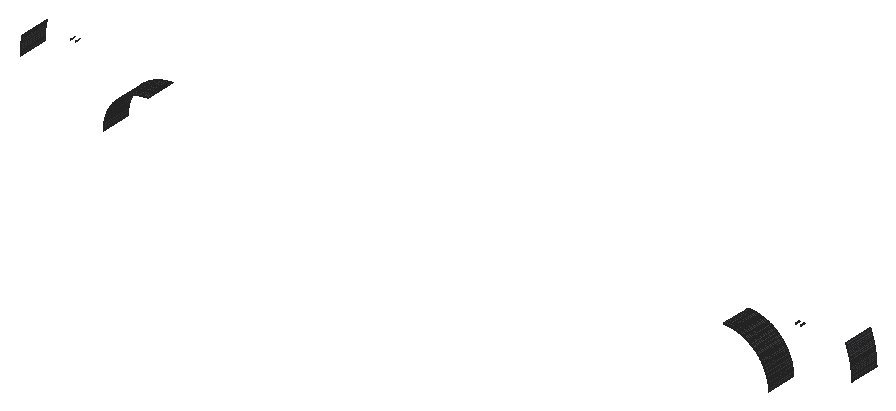
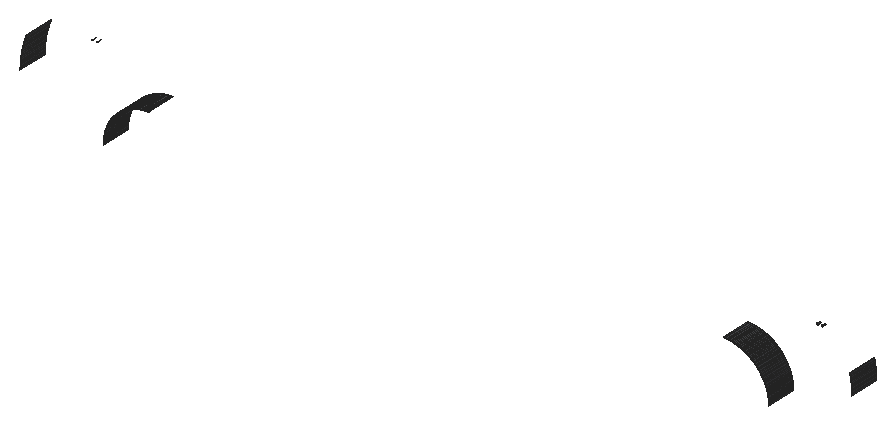
# SketchUp Ruby script. Lengths in inches.
U = 1.inch
M = Sketchup.active_model
def pt(a) = Geom::Point3d.new(a.map { |v| v * U })
def face(e, loops, mat)
  f = e.add_face(loops[0].map { |a| pt(a) })
  loops[1..].each { |l| e.add_face(l.map { |a| pt(a) }).erase! }
  f.material = f.back_material = mat if mat
  f
end
# faces: each face lists its corners as indices into pts; further lists are holes
def faces(e, pts, list, mat = nil) = list.each { |f| face(e, (f[0].is_a?(Array) ? f : [f]).map { |l| l.map { |i| pts[i] } }, mat) }
# xy, xz, yz: faces in a plane at the given z, y or x. An outline is a flat list of corners, or four numbers for a rectangle; further outlines are holes
def ring(l) = l.size == 4 ? [[l[0], l[1]], [l[2], l[1]], [l[2], l[3]], [l[0], l[3]]] : l.each_slice(2).to_a
def flat(e, list, mat, &to3) = list.each { |f| face(e, (f[0].is_a?(Array) ? f : [f]).map { |l| ring(l).map { |u, v| to3.(u, v) } }, mat) }
def xy(e, z, list, mat = nil) = flat(e, list, mat) { |x, y| [x, y, z] }
def xz(e, y, list, mat = nil) = flat(e, list, mat) { |x, z| [x, y, z] }
def yz(e, x, list, mat = nil) = flat(e, list, mat) { |y, z| [x, y, z] }
def lines(e, pts, list) = list.each { |a, b| e.add_line(pt(pts[a]), pt(pts[b])) }
# prism: a flat outline (further loops are holes) pulled along v
def prism(e, loops, v, mat = nil)
  f = face(e, loops, mat); d = Geom::Vector3d.new(v.map { |x| x * U })
  f.pushpull(f.normal.samedirection?(d) ? d.length : -d.length)
end
def box(e, o, s, mat = nil) = prism(e, [[o, [o[0] + s[0], o[1], o[2]], [o[0] + s[0], o[1] + s[1], o[2]], [o[0], o[1] + s[1], o[2]]]], [0, 0, s[2]], mat)
def at(x, y, z, deg = 0) = Geom::Transformation.translation(pt([x, y, z])) * Geom::Transformation.rotation(ORIGIN, Z_AXIS, deg.degrees)
def axes(o, x, y, z) = Geom::Transformation.new([*x, 0, *y, 0, *z, 0, *pt(o).to_a, 1])
def part(name) = M.definitions.add(name)
# library, detail: a bought-in or finely detailed component or shape, given as its bounding box
def library(name, o, s) = part(name).tap { |d| box(d.entities, o, s) }
def detail(e, o, s) = box(e.add_group.entities, o, s)
def put(e, d, t, mat = nil) = e.add_instance(d, t).tap { |i| i.material = mat if mat }
def group(e, t, mat = nil) = e.add_group.tap { |g| g.transformation = t; g.material = mat if mat }.entities
root = M.entities
M.materials.add("1432 AP 8245 TAR ROAD").color = [71, 72, 75]
M.materials.add("Outer Light").color = [251, 217, 152]
xy(root,563.79,[[293.53,95.37,293.76,107.37],[293.76,95.37,294,107.37],[522,95.37,522.2,107.37],[522.2,95.37,522.4,107.37]],"1432 AP 8245 TAR ROAD")
yz(root,243,[[95.37,560.79,107.37,561.07],[95.37,561.07,107.37,561.36]],"1432 AP 8245 TAR ROAD")
yz(root,276,[[95.37,545.79,107.37,546.03]],"1432 AP 8245 TAR ROAD")
yz(root,276.01,[[95.37,546.26,107.37,546.5]],"1432 AP 8245 TAR ROAD")
yz(root,540,[[95.37,545.79,107.37,545.99],[95.37,545.99,107.37,546.2]],"1432 AP 8245 TAR ROAD")
yz(root,573,[[95.37,560.79,107.37,561.07],[95.37,561.07,107.37,561.36]],"1432 AP 8245 TAR ROAD")
p = [[276,107.37,546.03],[276.01,107.37,546.26],[276.01,95.37,546.26],[276,95.37,546.03],[539.99,107.37,546.4],[540,107.37,546.2],
  [540,95.37,546.2],[539.99,95.37,546.4],[539.98,107.37,546.6],[539.98,95.37,546.6],[276.01,107.37,546.5],[276.02,107.37,546.73],
  [276.02,95.37,546.73],[276.01,95.37,546.5],[539.97,107.37,546.8],[539.97,95.37,546.8],[276.04,107.37,546.97],[276.04,95.37,546.97],
  [539.96,107.37,547],[539.96,95.37,547],[276.06,107.37,547.2],[276.06,95.37,547.2],[539.94,107.37,547.2],[539.94,95.37,547.2],
  [276.08,107.37,547.4375],[276.08,95.37,547.4375],[539.93,107.37,547.41],[539.93,95.37,547.41],[276.1,107.37,547.67],[276.1,95.37,547.67],
  [539.91,107.37,547.61],[539.91,95.37,547.61],[539.89,107.37,547.81],[539.89,95.37,547.81],[276.125,107.37,547.91],[276.125,95.37,547.91],
  [539.86,107.37,548.01],[539.86,95.37,548.01],[276.15,107.37,548.14],[276.15,95.37,548.14],[539.84,107.37,548.21],[539.84,95.37,548.21],
  [276.1875,107.37,548.375],[276.1875,95.37,548.375],[539.81,107.37,548.41],[539.81,95.37,548.41],[276.22,107.37,548.61],[276.22,95.37,548.61],
  [539.78,107.37,548.61],[539.78,95.37,548.61],[276.26,107.37,548.84],[276.26,95.37,548.84],[539.75,107.37,548.81],[539.75,95.37,548.81],
  [276.3,107.37,549.07],[276.3,95.37,549.07],[539.71,107.37,549.01],[539.71,95.37,549.01],[539.67,107.37,549.2],[539.67,95.37,549.2],
  [276.35,107.37,549.3],[276.35,95.37,549.3],[539.63,107.37,549.4],[539.63,95.37,549.4],[276.39,107.37,549.53],[276.39,95.37,549.53],
  [539.59,107.37,549.6],[539.59,95.37,549.6],[276.44,107.37,549.76],[276.44,95.37,549.76],[539.55,107.37,549.8],[539.55,95.37,549.8],
  [276.5,107.37,549.99],[276.5,95.37,549.99],[539.5,107.37,549.99],[539.5,95.37,549.99],[276.55,107.37,550.22],[276.55,95.37,550.22],
  [539.45,107.37,550.19],[539.45,95.37,550.19],[276.61,107.37,550.45],[276.61,95.37,550.45],[539.4,107.37,550.39],[539.4,95.37,550.39],
  [539.35,107.37,550.58],[539.35,95.37,550.58],[276.68,107.37,550.68],[276.68,95.37,550.68],[539.3,107.37,550.78],[539.3,95.37,550.78],
  [276.74,107.37,550.9],[276.74,95.37,550.9],[539.24,107.37,550.97],[539.24,95.37,550.97],[276.81,107.37,551.13],[276.81,95.37,551.13],
  [539.18,107.37,551.16],[539.18,95.37,551.16],[276.88,107.37,551.35],[276.88,95.37,551.35],[539.12,107.37,551.35],[539.12,95.37,551.35],
  [276.96,107.37,551.58],[276.96,95.37,551.58],[539.06,107.37,551.55],[539.06,95.37,551.55],[538.99,107.37,551.74],[538.99,95.37,551.74],
  [277.03,107.37,551.8],[277.03,95.37,551.8],[538.92,107.37,551.93],[538.92,95.37,551.93],[277.11,107.37,552.02],[277.11,95.37,552.02],
  [538.85,107.37,552.12],[538.85,95.37,552.12],[277.2,107.37,552.24],[277.2,95.37,552.24],[538.78,107.37,552.31],[538.78,95.37,552.31],
  [277.28,107.37,552.46],[277.28,95.37,552.46],[538.71,107.37,552.49],[538.71,95.37,552.49],[277.37,107.37,552.68],[277.37,95.37,552.68],
  [538.63,107.37,552.68],[538.63,95.37,552.68],[277.46,107.37,552.9],[277.46,95.37,552.9],[538.55,107.37,552.87],[538.55,95.37,552.87],
  [277.56,107.37,553.11],[277.56,95.37,553.11],[538.47,107.37,553.05],[538.47,95.37,553.05],[277.65,107.37,553.33],[277.65,95.37,553.33],
  [538.39,107.37,553.24],[538.39,95.37,553.24],[538.3,107.37,553.42],[538.3,95.37,553.42],[277.75,107.37,553.54],[277.75,95.37,553.54],
  [538.22,107.37,553.6],[538.22,95.37,553.6],[277.86,107.37,553.75],[277.86,95.37,553.75],[538.13,107.37,553.78],[538.13,95.37,553.78],
  [277.96,107.37,553.96],[277.96,95.37,553.96],[538.04,107.37,553.96],[538.04,95.37,553.96],[278.07,107.37,554.17],[278.07,95.37,554.17],
  [537.95,107.37,554.14],[537.95,95.37,554.14],[537.85,107.37,554.32],[537.85,95.37,554.32],[278.18,107.37,554.38],[278.18,95.37,554.38],
  [537.75,107.37,554.5],[537.75,95.37,554.5],[278.3,107.37,554.59],[278.3,95.37,554.59],[537.66,107.37,554.68],[537.66,95.37,554.68],
  [278.41,107.37,554.79],[278.41,95.37,554.79],[537.55,107.37,554.85],[537.55,95.37,554.85],[278.53,107.37,555],[278.53,95.37,555],
  [537.45,107.37,555.02],[537.45,95.37,555.02],[278.65,107.37,555.2],[278.65,95.37,555.2],[537.35,107.37,555.2],[537.35,95.37,555.2],
  [278.78,107.37,555.4],[278.78,95.37,555.4],[537.24,107.37,555.37],[537.24,95.37,555.37],[278.9,107.37,555.6],[278.9,95.37,555.6],
  [537.13,107.37,555.54],[537.13,95.37,555.54],[537.02,107.37,555.71],[537.02,95.37,555.71],[279.03,107.37,555.79],[279.03,95.37,555.79],
  [536.91,107.37,555.875],[536.91,95.37,555.875],[279.17,107.37,555.99],[279.17,95.37,555.99],[536.8,107.37,556.04],[536.8,95.37,556.04],
  [279.3,107.37,556.18],[279.3,95.37,556.18],[536.68,107.37,556.21],[536.68,95.37,556.21],[279.4375,107.37,556.37],[279.4375,95.37,556.37],
  [536.5625,107.37,556.37],[536.5625,95.37,556.37],[279.58,107.37,556.5625],[279.58,95.37,556.5625],[536.44,107.37,556.53],[536.44,95.37,556.53],
  [536.32,107.37,556.7],[536.32,95.37,556.7],[279.72,107.37,556.75],[279.72,95.37,556.75],[279.86,107.37,556.9375],[279.86,95.37,556.9375],
  [536.2,107.37,556.86],[536.2,95.37,556.86],[280.01,107.37,557.12],[280.01,95.37,557.12],[536.07,107.37,557.01],[536.07,95.37,557.01],
  [535.95,107.37,557.17],[535.95,95.37,557.17],[280.16,107.37,557.3],[280.16,95.37,557.3],[535.82,107.37,557.33],[535.82,95.37,557.33],
  [280.3125,107.37,557.48],[280.3125,95.37,557.48],[535.6875,107.37,557.48],[535.6875,95.37,557.48],[280.47,107.37,557.66],[280.47,95.37,557.66],
  [535.56,107.37,557.63],[535.56,95.37,557.63],[535.42,107.37,557.79],[535.42,95.37,557.79],[280.625,107.37,557.84],[280.625,95.37,557.84],
  [280.78,107.37,558.01],[280.78,95.37,558.01],[535.29,107.37,557.9375],[535.29,95.37,557.9375],[535.15,107.37,558.08],[535.15,95.37,558.08],
  [280.94,107.37,558.18],[280.94,95.37,558.18],[535.01,107.37,558.23],[535.01,95.37,558.23],[281.11,107.37,558.35],[281.11,95.37,558.35],
  [534.87,107.37,558.375],[534.87,95.37,558.375],[281.27,107.37,558.52],[281.27,95.37,558.52],[534.73,107.37,558.52],[534.73,95.37,558.52],
  [281.44,107.37,558.69],[281.44,95.37,558.69],[534.58,107.37,558.66],[534.58,95.37,558.66],[281.61,107.37,558.85],[281.61,95.37,558.85],
  [534.4375,107.37,558.8],[534.4375,95.37,558.8],[281.78,107.37,559.01],[281.78,95.37,559.01],[534.29,107.37,558.94],[534.29,95.37,558.94],
  [534.14,107.37,559.08],[534.14,95.37,559.08],[281.96,107.37,559.17],[281.96,95.37,559.17],[533.99,107.37,559.21],[533.99,95.37,559.21],
  [282.13,107.37,559.33],[282.13,95.37,559.33],[533.84,107.37,559.35],[533.84,95.37,559.35],[282.31,107.37,559.48],[282.31,95.37,559.48],
  [533.69,107.37,559.48],[533.69,95.37,559.48],[282.49,107.37,559.63],[282.49,95.37,559.63],[533.54,107.37,559.61],[533.54,95.37,559.61],
  [282.67,107.37,559.78],[282.67,95.37,559.78],[533.38,107.37,559.74],[533.38,95.37,559.74],[533.22,107.37,559.87],[533.22,95.37,559.87],
  [282.86,107.37,559.93],[282.86,95.37,559.93],[283.04,107.37,560.07],[283.04,95.37,560.07],[533.0625,107.37,559.99],[533.0625,95.37,559.99],
  [532.9,107.37,560.11],[532.9,95.37,560.11],[283.23,107.37,560.21],[283.23,95.37,560.21],[532.74,107.37,560.23],[532.74,95.37,560.23],
  [283.42,107.37,560.35],[283.42,95.37,560.35],[532.58,107.37,560.35],[532.58,95.37,560.35],[283.61,107.37,560.49],[283.61,95.37,560.49],
  [532.42,107.37,560.47],[532.42,95.37,560.47],[283.8,107.37,560.625],[283.8,95.37,560.625],[532.25,107.37,560.59],[532.25,95.37,560.59],
  [284,107.37,560.76],[284,95.37,560.76],[532.08,107.37,560.7],[532.08,95.37,560.7],[531.92,107.37,560.8125],[531.92,95.37,560.8125],
  [284.2,107.37,560.89],[284.2,95.37,560.89],[531.75,107.37,560.92],[531.75,95.37,560.92],[284.39,107.37,561.02],[284.39,95.37,561.02],
  [531.58,107.37,561.03],[531.58,95.37,561.03],[284.6,107.37,561.14],[284.6,95.37,561.14],[531.4,107.37,561.14],[531.4,95.37,561.14],
  [284.8,107.37,561.26],[284.8,95.37,561.26],[531.23,107.37,561.24],[531.23,95.37,561.24],[531.06,107.37,561.35],[531.06,95.37,561.35],
  [285,107.37,561.38],[285,95.37,561.38],[530.88,107.37,561.45],[530.88,95.37,561.45],[243.01,107.37,561.64],[243,107.37,561.36],
  [243,95.37,561.36],[243.01,95.37,561.64],[285.2,107.37,561.5],[285.2,95.37,561.5],[530.71,107.37,561.55],[530.71,95.37,561.55],
  [573,107.37,561.36],[572.99,107.37,561.64],[572.99,95.37,561.64],[573,95.37,561.36],[285.41,107.37,561.61],[285.41,95.37,561.61],
  [530.53,107.37,561.64],[530.53,95.37,561.64],[243.02,107.37,561.92],[243.02,95.37,561.92],[285.62,107.37,561.72],[285.62,95.37,561.72],
  [530.35,107.37,561.74],[530.35,95.37,561.74],[572.98,107.37,561.92],[572.98,95.37,561.92],[285.83,107.37,561.83],[285.83,95.37,561.83],
  [530.17,107.37,561.83],[530.17,95.37,561.83],[286.04,107.37,561.9375],[286.04,95.37,561.9375],[529.99,107.37,561.92],[529.99,95.37,561.92],
  [243.03,107.37,562.21],[243.03,95.37,562.21],[286.25,107.37,562.04],[286.25,95.37,562.04],[529.81,107.37,562.01],[529.81,95.37,562.01],
  [572.97,107.37,562.21],[572.97,95.37,562.21],[286.46,107.37,562.14],[286.46,95.37,562.14],[529.63,107.37,562.1],[529.63,95.37,562.1],
  [286.68,107.37,562.24],[286.68,95.37,562.24],[529.44,107.37,562.18],[529.44,95.37,562.18],[243.04,107.37,562.49],[243.04,95.37,562.49],
  [286.89,107.37,562.33],[286.89,95.37,562.33],[529.26,107.37,562.26],[529.26,95.37,562.26],[572.96,107.37,562.49],[572.96,95.37,562.49],
  [287.11,107.37,562.42],[287.11,95.37,562.42],[528.89,107.37,562.42],[529.07,107.37,562.34],[529.07,95.37,562.34],[528.89,95.37,562.42],
  [287.33,107.37,562.51],[287.33,95.37,562.51],[528.7,107.37,562.5],[528.7,95.37,562.5],[243.05,107.37,562.77],[243.05,95.37,562.77],
  [287.55,107.37,562.6],[287.55,95.37,562.6],[528.51,107.37,562.57],[528.51,95.37,562.57],[572.95,107.37,562.77],[572.95,95.37,562.77],
  [287.77,107.37,562.68],[287.77,95.37,562.68],[528.14,107.37,562.71],[528.32,107.37,562.64],[528.32,95.37,562.64],[528.14,95.37,562.71],
  [287.99,107.37,562.76],[287.99,95.37,562.76],[527.95,107.37,562.78],[527.95,95.37,562.78],[243.07,107.37,563.05],[243.07,95.37,563.05],
  [288.21,107.37,562.84],[288.21,95.37,562.84],[288.4375,107.37,562.91],[288.4375,95.37,562.91],[527.5625,107.37,562.91],[527.75,107.37,562.85],
  [527.75,95.37,562.85],[527.5625,95.37,562.91],[572.93,107.37,563.05],[572.93,95.37,563.05],[288.66,107.37,562.98],[288.66,95.37,562.98],
  [527.37,107.37,562.97],[527.37,95.37,562.97],[288.89,107.37,563.05],[288.89,95.37,563.05],[526.98,107.37,563.09],[527.18,107.37,563.03],
  [527.18,95.37,563.03],[526.98,95.37,563.09],[243.09,107.37,563.33],[243.09,95.37,563.33],[289.11,107.37,563.12],[289.11,95.37,563.12],
  [289.34,107.37,563.18],[289.34,95.37,563.18],[526.59,107.37,563.2],[526.79,107.37,563.14],[526.79,95.37,563.14],[526.59,95.37,563.2],
  [572.91,107.37,563.33],[572.91,95.37,563.33],[289.57,107.37,563.24],[289.57,95.37,563.24],[289.8,107.37,563.29],[289.8,95.37,563.29],
  [526.2,107.37,563.29],[526.4,107.37,563.25],[526.4,95.37,563.25],[526.2,95.37,563.29],[243.11,107.37,563.62],[243.11,95.37,563.62],
  [290.03,107.37,563.35],[290.03,95.37,563.35],[290.26,107.37,563.4],[290.26,95.37,563.4],[525.81,107.37,563.38],[526.01,107.37,563.34],
  [526.01,95.37,563.34],[525.81,95.37,563.38],[572.89,107.37,563.62],[572.89,95.37,563.62],[290.49,107.37,563.45],[290.49,95.37,563.45],
  [290.72,107.37,563.49],[290.72,95.37,563.49],[525.41,107.37,563.47],[525.61,107.37,563.43],[525.61,95.37,563.43],[525.41,95.37,563.47],
  [290.95,107.37,563.53],[290.95,95.37,563.53],[291.18,107.37,563.57],[291.18,95.37,563.57],[524.82,107.37,563.57],[525.02,107.37,563.54],
  [525.02,95.37,563.54],[524.82,95.37,563.57],[525.21,107.37,563.5],[525.21,95.37,563.5],[243.13,107.37,563.9],[243.13,95.37,563.9],
  [291.42,107.37,563.61],[291.42,95.37,563.61],[291.65,107.37,563.64],[291.65,95.37,563.64],[291.88,107.37,563.67],[291.88,95.37,563.67],
  [524.22,107.37,563.66],[524.42,107.37,563.63],[524.42,95.37,563.63],[524.22,95.37,563.66],[524.62,107.37,563.6],[524.62,95.37,563.6],
  [572.87,107.37,563.9],[572.87,95.37,563.9],[292.12,107.37,563.69],[292.12,95.37,563.69],[292.35,107.37,563.72],[292.35,95.37,563.72],
  [292.59,107.37,563.74],[292.59,95.37,563.74],[292.82,107.37,563.75],[292.82,95.37,563.75],[523.21,107.37,563.75],[523.41,107.37,563.74],
  [523.41,95.37,563.74],[523.21,95.37,563.75],[523.61,107.37,563.72],[523.61,95.37,563.72],[523.81,107.37,563.7],[523.81,95.37,563.7],
  [524.02,107.37,563.68],[524.02,95.37,563.68],[293.06,107.37,563.77],[293.06,95.37,563.77],[293.29,107.37,563.78],[293.29,95.37,563.78],
  [293.53,107.37,563.79],[293.53,95.37,563.79],[522.4,107.37,563.79],[522.61,107.37,563.78],[522.61,95.37,563.78],[522.4,95.37,563.79],
  [522.81,107.37,563.77],[522.81,95.37,563.77],[523.01,107.37,563.76],[523.01,95.37,563.76],[243.16,107.37,564.18],[243.16,95.37,564.18],
  [572.84,107.37,564.18],[572.84,95.37,564.18],[243.1875,107.37,564.46],[243.1875,95.37,564.46],[572.8125,107.37,564.46],[572.8125,95.37,564.46],
  [243.22,107.37,564.74],[243.22,95.37,564.74],[572.78,107.37,564.74],[572.78,95.37,564.74],[243.25,107.37,565.02],[243.25,95.37,565.02],
  [572.75,107.37,565.02],[572.75,95.37,565.02],[243.28,107.37,565.3],[243.28,95.37,565.3],[572.72,107.37,565.3],[572.72,95.37,565.3],
  [243.32,107.37,565.58],[243.32,95.37,565.58],[572.68,107.37,565.58],[572.68,95.37,565.58],[243.36,107.37,565.86],[243.36,95.37,565.86],
  [572.64,107.37,565.86],[572.64,95.37,565.86],[243.4,107.37,566.14],[243.4,95.37,566.14],[572.6,107.37,566.14],[572.6,95.37,566.14],
  [243.44,107.37,566.42],[243.44,95.37,566.42],[572.56,107.37,566.42],[572.56,95.37,566.42],[243.49,107.37,566.7],[243.49,95.37,566.7],
  [572.51,107.37,566.7],[572.51,95.37,566.7],[243.54,107.37,566.98],[243.54,95.37,566.98],[572.46,107.37,566.98],[572.46,95.37,566.98],
  [243.59,107.37,567.26],[243.59,95.37,567.26],[572.41,107.37,567.26],[572.41,95.37,567.26],[243.64,107.37,567.54],[243.64,95.37,567.54],
  [572.36,107.37,567.54],[572.36,95.37,567.54],[243.69,107.37,567.82],[243.69,95.37,567.82],[572.31,107.37,567.82],[572.31,95.37,567.82],
  [243.75,107.37,568.09],[243.75,95.37,568.09],[572.25,107.37,568.09],[572.25,95.37,568.09],[243.81,107.37,568.37],[243.81,95.37,568.37],
  [572.19,107.37,568.37],[572.19,95.37,568.37],[243.87,107.37,568.65],[243.87,95.37,568.65],[572.13,107.37,568.65],[572.13,95.37,568.65],
  [572.07,107.37,568.92],[572.07,95.37,568.92],[572.01,107.37,569.2],[572.01,95.37,569.2],[571.9375,107.37,569.47],[571.9375,95.37,569.47],
  [571.87,107.37,569.74],[571.87,95.37,569.74],[571.8,107.37,570.02],[571.8,95.37,570.02],[571.72,107.37,570.29],[571.72,95.37,570.29],
  [571.65,107.37,570.5625],[571.65,95.37,570.5625],[571.57,107.37,570.84],[571.57,95.37,570.84],[571.49,107.37,571.11],[571.49,95.37,571.11],
  [571.41,107.37,571.38],[571.41,95.37,571.38],[571.32,107.37,571.65],[571.32,95.37,571.65],[571.24,107.37,571.92],[571.24,95.37,571.92],
  [571.15,107.37,572.19],[571.15,95.37,572.19],[571.06,107.37,572.45],[571.06,95.37,572.45],[570.97,107.37,572.72],[570.97,95.37,572.72],
  [570.87,107.37,572.99],[570.87,95.37,572.99],[570.77,107.37,573.25],[570.77,95.37,573.25],[570.68,107.37,573.52],[570.68,95.37,573.52],
  [570.58,107.37,573.78],[570.58,95.37,573.78],[263.2,95.37,573.86],[263.1,95.37,573.73],[263.1,96.87,573.73],[263.2,96.87,573.86],
  [263.2,96.87,573.86],[263.1,96.87,573.73],[263.1,95.37,573.73],[263.2,95.37,573.86],[265.05,95.37,573.6875],[265.15,95.37,573.8],
  [265.15,96.87,573.8],[265.05,96.87,573.6875],[265.05,96.87,573.6875],[265.15,96.87,573.8],[265.15,95.37,573.8],[265.05,95.37,573.6875],
  [550.85,95.37,573.8],[550.95,95.37,573.6875],[550.95,96.87,573.6875],[550.85,96.87,573.8],[550.85,96.87,573.8],[550.95,96.87,573.6875],
  [550.95,95.37,573.6875],[550.85,95.37,573.8],[552.9,95.37,573.73],[552.8,95.37,573.86],[552.8,96.87,573.86],[552.9,96.87,573.73],
  [552.9,96.87,573.73],[552.8,96.87,573.86],[552.8,95.37,573.86],[552.9,95.37,573.73],[265.25,95.37,573.91],[265.25,96.87,573.91],
  [265.25,96.87,573.91],[265.25,95.37,573.91],[550.75,95.37,573.91],[550.75,96.87,573.91],[550.75,96.87,573.91],[550.75,95.37,573.91],
  [570.47,107.37,574.04],[570.47,95.37,574.04],[263.31,95.37,573.98],[263.31,96.87,573.98],[263.31,96.87,573.98],[263.31,95.37,573.98],
  [265.36,95.37,574.01],[265.36,96.87,574.01],[265.36,96.87,574.01],[265.36,95.37,574.01],[550.64,95.37,574.01],[550.64,96.87,574.01],
  [550.64,96.87,574.01],[550.64,95.37,574.01],[552.69,95.37,573.98],[552.69,96.87,573.98],[552.69,96.87,573.98],[552.69,95.37,573.98],
  [263.41,95.37,574.11],[263.41,96.87,574.11],[263.41,96.87,574.11],[263.41,95.37,574.11],[265.46,95.37,574.12],[265.46,96.87,574.12],
  [265.46,96.87,574.12],[265.46,95.37,574.12],[550.54,95.37,574.12],[550.54,96.87,574.12],[550.54,96.87,574.12],[550.54,95.37,574.12],
  [552.59,95.37,574.11],[552.59,96.87,574.11],[552.59,96.87,574.11],[552.59,95.37,574.11]]
faces(root,p,[[0,1,2,3],[4,5,6,7],[8,4,7,9],[10,11,12,13],[14,8,9,15],[11,16,17,12],[18,14,15,19],[16,20,21,17],
  [22,18,19,23],[20,24,25,21],[26,22,23,27],[24,28,29,25],[30,26,27,31],[32,30,31,33],[28,34,35,29],[36,32,33,37],
  [34,38,39,35],[40,36,37,41],[38,42,43,39],[44,40,41,45],[42,46,47,43],[48,44,45,49],[46,50,51,47],[52,48,49,53],
  [50,54,55,51],[56,52,53,57],[58,56,57,59],[54,60,61,55],[62,58,59,63],[60,64,65,61],[66,62,63,67],[64,68,69,65],
  [70,66,67,71],[68,72,73,69],[74,70,71,75],[72,76,77,73],[78,74,75,79],[76,80,81,77],[82,78,79,83],[84,82,83,85],
  [80,86,87,81],[88,84,85,89],[86,90,91,87],[92,88,89,93],[90,94,95,91],[96,92,93,97],[94,98,99,95],[100,96,97,101],
  [98,102,103,99],[104,100,101,105],[106,104,105,107],[102,108,109,103],[110,106,107,111],[108,112,113,109],[114,110,111,115],[112,116,117,113],
  [118,114,115,119],[116,120,121,117],[122,118,119,123],[120,124,125,121],[126,122,123,127],[124,128,129,125],[130,126,127,131],[128,132,133,129],
  [134,130,131,135],[132,136,137,133],[138,134,135,139],[140,138,139,141],[136,142,143,137],[144,140,141,145],[142,146,147,143],[148,144,145,149],
  [146,150,151,147],[152,148,149,153],[150,154,155,151],[156,152,153,157],[158,156,157,159],[154,160,161,155],[162,158,159,163],[160,164,165,161],
  [166,162,163,167],[164,168,169,165],[170,166,167,171],[168,172,173,169],[174,170,171,175],[172,176,177,173],[178,174,175,179],[176,180,181,177],
  [182,178,179,183],[180,184,185,181],[186,182,183,187],[188,186,187,189],[184,190,191,185],[192,188,189,193],[190,194,195,191],[196,192,193,197],
  [194,198,199,195],[200,196,197,201],[198,202,203,199],[204,200,201,205],[202,206,207,203],[208,204,205,209],[210,208,209,211],[206,212,213,207],
  [212,214,215,213],[216,210,211,217],[214,218,219,215],[220,216,217,221],[222,220,221,223],[218,224,225,219],[226,222,223,227],[224,228,229,225],
  [230,226,227,231],[228,232,233,229],[234,230,231,235],[236,234,235,237],[232,238,239,233],[238,240,241,239],[242,236,237,243],[244,242,243,245],
  [240,246,247,241],[248,244,245,249],[246,250,251,247],[252,248,249,253],[250,254,255,251],[256,252,253,257],[254,258,259,255],[260,256,257,261],
  [258,262,263,259],[264,260,261,265],[262,266,267,263],[268,264,265,269],[270,268,269,271],[266,272,273,267],[274,270,271,275],[272,276,277,273],
  [278,274,275,279],[276,280,281,277],[282,278,279,283],[280,284,285,281],[286,282,283,287],[284,288,289,285],[290,286,287,291],[292,290,291,293],
  [288,294,295,289],[294,296,297,295],[298,292,293,299],[300,298,299,301],[296,302,303,297],[304,300,301,305],[302,306,307,303],[308,304,305,309],
  [306,310,311,307],[312,308,309,313],[310,314,315,311],[316,312,313,317],[314,318,319,315],[320,316,317,321],[322,320,321,323],[318,324,325,319],
  [326,322,323,327],[324,328,329,325],[330,326,327,331],[328,332,333,329],[334,330,331,335],[332,336,337,333],[338,334,335,339],[340,338,339,341],
  [336,342,343,337],[344,340,341,345],[346,347,348,349],[342,350,351,343],[352,344,345,353],[354,355,356,357],[350,358,359,351],[360,352,353,361],
  [362,346,349,363],[358,364,365,359],[366,360,361,367],[355,368,369,356],[364,370,371,365],[372,366,367,373],[370,374,375,371],[376,372,373,377],
  [378,362,363,379],[374,380,381,375],[382,376,377,383],[368,384,385,369],[380,386,387,381],[388,382,383,389],[386,390,391,387],[392,388,389,393],
  [394,378,379,395],[390,396,397,391],[398,392,393,399],[384,400,401,385],[396,402,403,397],[404,405,406,407],[405,398,399,406],[402,408,409,403],
  [410,404,407,411],[412,394,395,413],[408,414,415,409],[416,410,411,417],[400,418,419,401],[414,420,421,415],[422,423,424,425],[423,416,417,424],
  [420,426,427,421],[428,422,425,429],[430,412,413,431],[426,432,433,427],[432,434,435,433],[436,437,438,439],[437,428,429,438],[418,440,441,419],
  [434,442,443,435],[444,436,439,445],[442,446,447,443],[448,449,450,451],[449,444,445,450],[452,430,431,453],[446,454,455,447],[454,456,457,455],
  [458,459,460,461],[459,448,451,460],[440,462,463,441],[456,464,465,457],[464,466,467,465],[468,469,470,471],[469,458,461,470],[472,452,453,473],
  [466,474,475,467],[474,476,477,475],[478,479,480,481],[479,468,471,480],[462,482,483,463],[476,484,485,477],[484,486,487,485],[488,489,490,491],
  [489,478,481,490],[486,492,493,487],[492,494,495,493],[496,497,498,499],[497,500,501,498],[500,488,491,501],[502,472,473,503],[494,504,505,495],
  [504,506,507,505],[506,508,509,507],[510,511,512,513],[511,514,515,512],[514,496,499,515],[482,516,517,483],[508,518,519,509],[518,520,521,519],
  [520,522,523,521],[522,524,525,523],[526,527,528,529],[527,530,531,528],[530,532,533,531],[532,534,535,533],[534,510,513,535],[524,536,537,525],
  [536,538,539,537],[538,540,541,539],[542,543,544,545],[543,546,547,544],[546,548,549,547],[548,526,529,549],[550,502,503,551],[516,552,553,517],
  [554,550,551,555],[552,556,557,553],[558,554,555,559],[556,560,561,557],[562,558,559,563],[560,564,565,561],[566,562,563,567],[564,568,569,565],
  [570,566,567,571],[568,572,573,569],[574,570,571,575],[572,576,577,573],[578,574,575,579],[576,580,581,577],[582,578,579,583],[580,584,585,581],
  [586,582,583,587],[584,588,589,585],[590,586,587,591],[588,592,593,589],[594,590,591,595],[592,596,597,593],[598,594,595,599],[596,600,601,597],
  [602,598,599,603],[600,604,605,601],[606,602,603,607],[604,608,609,605],[610,606,607,611],[608,612,613,609],[614,610,611,615],[612,616,617,613],
  [616,618,619,617],[618,620,621,619],[620,622,623,621],[622,624,625,623],[624,626,627,625],[626,628,629,627],[628,630,631,629],[630,632,633,631],
  [632,634,635,633],[634,636,637,635],[636,638,639,637],[638,640,641,639],[640,642,643,641],[642,644,645,643],[644,646,647,645],[646,648,649,647],
  [648,650,651,649],[650,652,653,651],[652,654,655,653],[656,657,658,659],[664,665,666,667],[672,673,674,675],[680,681,682,683],[665,688,689,666],
  [692,672,675,693],[654,696,697,655],[698,656,659,699],[688,702,703,689],[706,692,693,707],[681,710,711,682],[714,698,699,715],[702,718,719,703],
  [722,706,707,723],[710,726,727,711]],"1432 AP 8245 TAR ROAD")
faces(root,p,[[660,661,662,663],[668,669,670,671],[676,677,678,679],[684,685,686,687],[669,690,691,670],[694,676,679,695],[700,660,663,701],[690,704,705,691],
  [708,694,695,709],[685,712,713,686],[716,700,701,717],[704,720,721,705],[724,708,709,725],[712,728,729,713]],"Outer Light")
